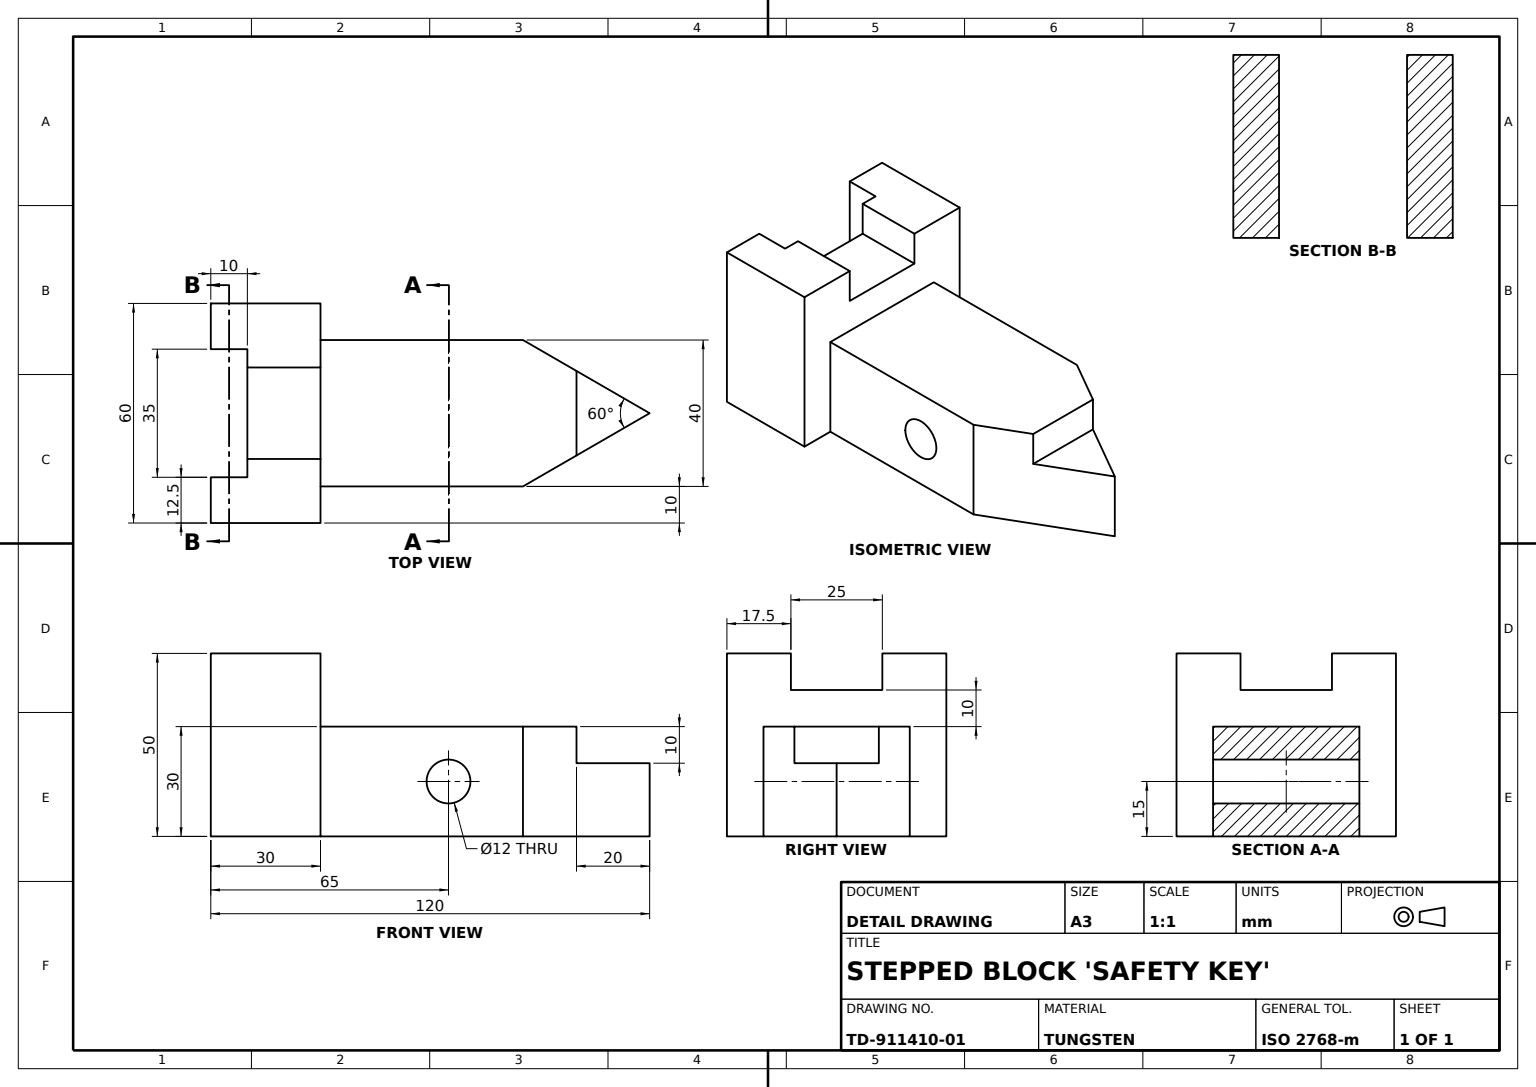
ISO-10303-21;
HEADER;
FILE_DESCRIPTION((''),'2;1');
FILE_NAME('','',(''),(''),'','','');
FILE_SCHEMA(('AUTOMOTIVE_DESIGN'));
ENDSEC;
DATA;
#1=APPLICATION_CONTEXT('');
#2=PRODUCT_CONTEXT('',#1,'mechanical');
#3=PRODUCT('','','',(#2));
#4=PRODUCT_DEFINITION_FORMATION('','',#3);
#5=PRODUCT_DEFINITION_CONTEXT('',#1,'design');
#6=PRODUCT_DEFINITION('','',#4,#5);
#7=PRODUCT_DEFINITION_SHAPE('','',#6);
#8=(LENGTH_UNIT()NAMED_UNIT(*)SI_UNIT(.MILLI.,.METRE.));
#9=(NAMED_UNIT(*)PLANE_ANGLE_UNIT()SI_UNIT($,.RADIAN.));
#10=(NAMED_UNIT(*)SI_UNIT($,.STERADIAN.)SOLID_ANGLE_UNIT());
#11=UNCERTAINTY_MEASURE_WITH_UNIT(LENGTH_MEASURE(0.005),#8,'distance_accuracy_value','');
#12=(GEOMETRIC_REPRESENTATION_CONTEXT(3)GLOBAL_UNCERTAINTY_ASSIGNED_CONTEXT((#11))GLOBAL_UNIT_ASSIGNED_CONTEXT((#8,#9,#10))REPRESENTATION_CONTEXT('',''));
#13=CARTESIAN_POINT('',(-5.,17.5,50.));
#14=VERTEX_POINT('',#13);
#15=CARTESIAN_POINT('',(-15.,17.5,50.));
#16=VERTEX_POINT('',#15);
#17=CARTESIAN_POINT('',(0.,17.5,50.));
#18=DIRECTION('',(-1.,0.,0.));
#19=VECTOR('',#18,1000.);
#20=LINE('',#17,#19);
#21=EDGE_CURVE('',#14,#16,#20,.T.);
#22=ORIENTED_EDGE('',*,*,#21,.F.);
#23=CARTESIAN_POINT('',(-5.,12.5,50.));
#24=VERTEX_POINT('',#23);
#25=CARTESIAN_POINT('',(-5.,0.,50.));
#26=DIRECTION('',(0.,1.,0.));
#27=VECTOR('',#26,1000.);
#28=LINE('',#25,#27);
#29=EDGE_CURVE('',#24,#14,#28,.T.);
#30=ORIENTED_EDGE('',*,*,#29,.F.);
#31=CARTESIAN_POINT('',(15.,12.5,50.));
#32=VERTEX_POINT('',#31);
#33=CARTESIAN_POINT('',(-30.,12.5,50.));
#34=DIRECTION('',(1.,0.,0.));
#35=VECTOR('',#34,1000.);
#36=LINE('',#33,#35);
#37=EDGE_CURVE('',#24,#32,#36,.T.);
#38=ORIENTED_EDGE('',*,*,#37,.T.);
#39=CARTESIAN_POINT('',(15.,30.,50.));
#40=VERTEX_POINT('',#39);
#41=CARTESIAN_POINT('',(15.,-30.,50.));
#42=LINE('',#41,#27);
#43=EDGE_CURVE('',#32,#40,#42,.T.);
#44=ORIENTED_EDGE('',*,*,#43,.T.);
#45=CARTESIAN_POINT('',(-15.,30.,50.));
#46=VERTEX_POINT('',#45);
#47=LINE('',#39,#19);
#48=EDGE_CURVE('',#40,#46,#47,.T.);
#49=ORIENTED_EDGE('',*,*,#48,.T.);
#50=DIRECTION('',(0.,-1.,0.));
#51=VECTOR('',#50,1000.);
#52=LINE('',#45,#51);
#53=EDGE_CURVE('',#46,#16,#52,.T.);
#54=ORIENTED_EDGE('',*,*,#53,.T.);
#55=EDGE_LOOP('',(#22,#30,#38,#44,#49,#54));
#56=FACE_BOUND('',#55,.T.);
#57=CARTESIAN_POINT('',(0.,0.,50.));
#58=DIRECTION('',(0.,0.,1.));
#59=AXIS2_PLACEMENT_3D('',#57,#58,#34);
#60=PLANE('',#59);
#61=ADVANCED_FACE('',(#56),#60,.T.);
#62=VERTEX_POINT('',#41);
#63=CARTESIAN_POINT('',(15.,-30.,0.));
#64=VERTEX_POINT('',#63);
#65=DIRECTION('',(0.,0.,-1.));
#66=VECTOR('',#65,1000.);
#67=LINE('',#41,#66);
#68=EDGE_CURVE('',#62,#64,#67,.T.);
#69=ORIENTED_EDGE('',*,*,#68,.F.);
#70=CARTESIAN_POINT('',(-15.,-30.,50.));
#71=VERTEX_POINT('',#70);
#72=LINE('',#70,#35);
#73=EDGE_CURVE('',#71,#62,#72,.T.);
#74=ORIENTED_EDGE('',*,*,#73,.F.);
#75=CARTESIAN_POINT('',(-15.,-30.,0.));
#76=VERTEX_POINT('',#75);
#77=LINE('',#70,#66);
#78=EDGE_CURVE('',#71,#76,#77,.T.);
#79=ORIENTED_EDGE('',*,*,#78,.T.);
#80=LINE('',#75,#35);
#81=EDGE_CURVE('',#76,#64,#80,.T.);
#82=ORIENTED_EDGE('',*,*,#81,.T.);
#83=EDGE_LOOP('',(#69,#74,#79,#82));
#84=FACE_BOUND('',#83,.T.);
#85=AXIS2_PLACEMENT_3D('',#70,#26,#58);
#86=PLANE('',#85);
#87=ADVANCED_FACE('',(#84),#86,.F.);
#88=CARTESIAN_POINT('',(-15.,-17.5,0.));
#89=VERTEX_POINT('',#88);
#90=CARTESIAN_POINT('',(-15.,30.,0.));
#91=LINE('',#90,#51);
#92=EDGE_CURVE('',#89,#76,#91,.T.);
#93=ORIENTED_EDGE('',*,*,#92,.T.);
#94=ORIENTED_EDGE('',*,*,#78,.F.);
#95=CARTESIAN_POINT('',(-15.,-17.5,50.));
#96=VERTEX_POINT('',#95);
#97=EDGE_CURVE('',#96,#71,#52,.T.);
#98=ORIENTED_EDGE('',*,*,#97,.F.);
#99=CARTESIAN_POINT('',(-15.,-17.5,62.));
#100=LINE('',#99,#66);
#101=EDGE_CURVE('',#96,#89,#100,.T.);
#102=ORIENTED_EDGE('',*,*,#101,.T.);
#103=EDGE_LOOP('',(#93,#94,#98,#102));
#104=FACE_BOUND('',#103,.T.);
#105=AXIS2_PLACEMENT_3D('',#45,#34,#65);
#106=PLANE('',#105);
#107=ADVANCED_FACE('',(#104),#106,.F.);
#108=CARTESIAN_POINT('',(44.,-20.,15.));
#109=VERTEX_POINT('',#108);
#110=CARTESIAN_POINT('',(50.,-20.,15.));
#111=AXIS2_PLACEMENT_3D('',#110,#26,#18);
#112=CIRCLE('',#111,6.);
#113=EDGE_CURVE('',#109,#109,#112,.T.);
#114=ORIENTED_EDGE('',*,*,#113,.F.);
#115=EDGE_LOOP('',(#114));
#116=FACE_BOUND('',#115,.T.);
#117=CARTESIAN_POINT('',(44.,20.,15.));
#118=VERTEX_POINT('',#117);
#119=CARTESIAN_POINT('',(50.,20.,15.));
#120=AXIS2_PLACEMENT_3D('',#119,#26,#18);
#121=CIRCLE('',#120,6.);
#122=EDGE_CURVE('',#118,#118,#121,.T.);
#123=ORIENTED_EDGE('',*,*,#122,.T.);
#124=EDGE_LOOP('',(#123));
#125=FACE_BOUND('',#124,.T.);
#126=CYLINDRICAL_SURFACE('',#111,6.);
#127=ADVANCED_FACE('',(#116,#125),#126,.F.);
#128=CARTESIAN_POINT('',(15.,20.,0.));
#129=VERTEX_POINT('',#128);
#130=CARTESIAN_POINT('',(70.358984,20.,0.));
#131=VERTEX_POINT('',#130);
#132=LINE('',#128,#35);
#133=EDGE_CURVE('',#129,#131,#132,.T.);
#134=ORIENTED_EDGE('',*,*,#133,.F.);
#135=CARTESIAN_POINT('',(15.,20.,30.));
#136=VERTEX_POINT('',#135);
#137=LINE('',#135,#66);
#138=EDGE_CURVE('',#136,#129,#137,.T.);
#139=ORIENTED_EDGE('',*,*,#138,.F.);
#140=CARTESIAN_POINT('',(70.358984,20.,30.));
#141=VERTEX_POINT('',#140);
#142=LINE('',#135,#35);
#143=EDGE_CURVE('',#136,#141,#142,.T.);
#144=ORIENTED_EDGE('',*,*,#143,.T.);
#145=CARTESIAN_POINT('',(70.358984,20.,62.));
#146=LINE('',#145,#66);
#147=EDGE_CURVE('',#141,#131,#146,.T.);
#148=ORIENTED_EDGE('',*,*,#147,.T.);
#149=EDGE_LOOP('',(#134,#139,#144,#148));
#150=FACE_BOUND('',#149,.T.);
#151=ORIENTED_EDGE('',*,*,#122,.F.);
#152=EDGE_LOOP('',(#151));
#153=FACE_BOUND('',#152,.T.);
#154=AXIS2_PLACEMENT_3D('',#135,#26,#18);
#155=PLANE('',#154);
#156=ADVANCED_FACE('',(#150,#153),#155,.T.);
#157=CARTESIAN_POINT('',(15.,30.,0.));
#158=VERTEX_POINT('',#157);
#159=LINE('',#39,#66);
#160=EDGE_CURVE('',#40,#158,#159,.T.);
#161=ORIENTED_EDGE('',*,*,#160,.T.);
#162=VERTEX_POINT('',#90);
#163=LINE('',#157,#19);
#164=EDGE_CURVE('',#158,#162,#163,.T.);
#165=ORIENTED_EDGE('',*,*,#164,.T.);
#166=LINE('',#45,#66);
#167=EDGE_CURVE('',#46,#162,#166,.T.);
#168=ORIENTED_EDGE('',*,*,#167,.F.);
#169=ORIENTED_EDGE('',*,*,#48,.F.);
#170=EDGE_LOOP('',(#161,#165,#168,#169));
#171=FACE_BOUND('',#170,.T.);
#172=AXIS2_PLACEMENT_3D('',#39,#50,#65);
#173=PLANE('',#172);
#174=ADVANCED_FACE('',(#171),#173,.F.);
#175=ORIENTED_EDGE('',*,*,#143,.F.);
#176=CARTESIAN_POINT('',(15.,-20.,30.));
#177=VERTEX_POINT('',#176);
#178=LINE('',#176,#27);
#179=EDGE_CURVE('',#177,#136,#178,.T.);
#180=ORIENTED_EDGE('',*,*,#179,.F.);
#181=CARTESIAN_POINT('',(70.358984,-20.,30.));
#182=VERTEX_POINT('',#181);
#183=CARTESIAN_POINT('',(105.,-20.,30.));
#184=LINE('',#183,#19);
#185=EDGE_CURVE('',#182,#177,#184,.T.);
#186=ORIENTED_EDGE('',*,*,#185,.F.);
#187=CARTESIAN_POINT('',(85.,-11.547005,30.));
#188=VERTEX_POINT('',#187);
#189=CARTESIAN_POINT('',(26.25,-45.466334,30.));
#190=DIRECTION('',(-0.866025404,-0.5,0.));
#191=VECTOR('',#190,1000.);
#192=LINE('',#189,#191);
#193=EDGE_CURVE('',#188,#182,#192,.T.);
#194=ORIENTED_EDGE('',*,*,#193,.F.);
#195=CARTESIAN_POINT('',(85.,11.547005,30.));
#196=VERTEX_POINT('',#195);
#197=CARTESIAN_POINT('',(85.,0.,30.));
#198=LINE('',#197,#51);
#199=EDGE_CURVE('',#196,#188,#198,.T.);
#200=ORIENTED_EDGE('',*,*,#199,.F.);
#201=CARTESIAN_POINT('',(26.25,45.466334,30.));
#202=DIRECTION('',(-0.866025404,0.5,0.));
#203=VECTOR('',#202,1000.);
#204=LINE('',#201,#203);
#205=EDGE_CURVE('',#196,#141,#204,.T.);
#206=ORIENTED_EDGE('',*,*,#205,.T.);
#207=EDGE_LOOP('',(#175,#180,#186,#194,#200,#206));
#208=FACE_BOUND('',#207,.T.);
#209=CARTESIAN_POINT('',(0.,0.,30.));
#210=AXIS2_PLACEMENT_3D('',#209,#65,#18);
#211=PLANE('',#210);
#212=ADVANCED_FACE('',(#208),#211,.F.);
#213=CARTESIAN_POINT('',(70.358984,-20.,0.));
#214=VERTEX_POINT('',#213);
#215=CARTESIAN_POINT('',(70.358984,-20.,62.));
#216=LINE('',#215,#66);
#217=EDGE_CURVE('',#182,#214,#216,.T.);
#218=ORIENTED_EDGE('',*,*,#217,.F.);
#219=ORIENTED_EDGE('',*,*,#185,.T.);
#220=CARTESIAN_POINT('',(15.,-20.,0.));
#221=VERTEX_POINT('',#220);
#222=LINE('',#176,#66);
#223=EDGE_CURVE('',#177,#221,#222,.T.);
#224=ORIENTED_EDGE('',*,*,#223,.T.);
#225=CARTESIAN_POINT('',(105.,-20.,0.));
#226=LINE('',#225,#19);
#227=EDGE_CURVE('',#214,#221,#226,.T.);
#228=ORIENTED_EDGE('',*,*,#227,.F.);
#229=EDGE_LOOP('',(#218,#219,#224,#228));
#230=FACE_BOUND('',#229,.T.);
#231=ORIENTED_EDGE('',*,*,#113,.T.);
#232=EDGE_LOOP('',(#231));
#233=FACE_BOUND('',#232,.T.);
#234=AXIS2_PLACEMENT_3D('',#183,#50,#34);
#235=PLANE('',#234);
#236=ADVANCED_FACE('',(#230,#233),#235,.T.);
#237=CARTESIAN_POINT('',(85.,-11.547005,20.));
#238=VERTEX_POINT('',#237);
#239=CARTESIAN_POINT('',(85.,-11.547005,62.));
#240=VECTOR('',#58,1000.);
#241=LINE('',#239,#240);
#242=EDGE_CURVE('',#238,#188,#241,.T.);
#243=ORIENTED_EDGE('',*,*,#242,.F.);
#244=CARTESIAN_POINT('',(85.,11.547005,20.));
#245=VERTEX_POINT('',#244);
#246=CARTESIAN_POINT('',(85.,15.,20.));
#247=LINE('',#246,#51);
#248=EDGE_CURVE('',#238,#245,#247,.F.);
#249=ORIENTED_EDGE('',*,*,#248,.T.);
#250=CARTESIAN_POINT('',(85.,11.547005,62.));
#251=LINE('',#250,#240);
#252=EDGE_CURVE('',#245,#196,#251,.T.);
#253=ORIENTED_EDGE('',*,*,#252,.T.);
#254=ORIENTED_EDGE('',*,*,#199,.T.);
#255=EDGE_LOOP('',(#243,#249,#253,#254));
#256=FACE_BOUND('',#255,.T.);
#257=CARTESIAN_POINT('',(85.,15.,44.));
#258=AXIS2_PLACEMENT_3D('',#257,#34,#65);
#259=PLANE('',#258);
#260=ADVANCED_FACE('',(#256),#259,.T.);
#261=ORIENTED_EDGE('',*,*,#101,.F.);
#262=CARTESIAN_POINT('',(-5.,-17.5,50.));
#263=VERTEX_POINT('',#262);
#264=CARTESIAN_POINT('',(0.,-17.5,50.));
#265=LINE('',#264,#35);
#266=EDGE_CURVE('',#96,#263,#265,.T.);
#267=ORIENTED_EDGE('',*,*,#266,.T.);
#268=CARTESIAN_POINT('',(-5.,-17.5,0.));
#269=VERTEX_POINT('',#268);
#270=CARTESIAN_POINT('',(-5.,-17.5,62.));
#271=LINE('',#270,#66);
#272=EDGE_CURVE('',#269,#263,#271,.F.);
#273=ORIENTED_EDGE('',*,*,#272,.F.);
#274=CARTESIAN_POINT('',(0.,-17.5,0.));
#275=LINE('',#274,#19);
#276=EDGE_CURVE('',#269,#89,#275,.T.);
#277=ORIENTED_EDGE('',*,*,#276,.T.);
#278=EDGE_LOOP('',(#261,#267,#273,#277));
#279=FACE_BOUND('',#278,.T.);
#280=AXIS2_PLACEMENT_3D('',#270,#50,#65);
#281=PLANE('',#280);
#282=ADVANCED_FACE('',(#279),#281,.F.);
#283=CARTESIAN_POINT('',(-15.,17.5,0.));
#284=VERTEX_POINT('',#283);
#285=CARTESIAN_POINT('',(-5.,17.5,0.));
#286=VERTEX_POINT('',#285);
#287=CARTESIAN_POINT('',(0.,17.5,0.));
#288=LINE('',#287,#35);
#289=EDGE_CURVE('',#284,#286,#288,.T.);
#290=ORIENTED_EDGE('',*,*,#289,.T.);
#291=CARTESIAN_POINT('',(-5.,17.5,62.));
#292=LINE('',#291,#66);
#293=EDGE_CURVE('',#286,#14,#292,.F.);
#294=ORIENTED_EDGE('',*,*,#293,.T.);
#295=ORIENTED_EDGE('',*,*,#21,.T.);
#296=CARTESIAN_POINT('',(-15.,17.5,62.));
#297=LINE('',#296,#66);
#298=EDGE_CURVE('',#16,#284,#297,.T.);
#299=ORIENTED_EDGE('',*,*,#298,.T.);
#300=EDGE_LOOP('',(#290,#294,#295,#299));
#301=FACE_BOUND('',#300,.T.);
#302=AXIS2_PLACEMENT_3D('',#296,#26,#58);
#303=PLANE('',#302);
#304=ADVANCED_FACE('',(#301),#303,.F.);
#305=CARTESIAN_POINT('',(15.,12.5,40.));
#306=VERTEX_POINT('',#305);
#307=LINE('',#31,#240);
#308=EDGE_CURVE('',#306,#32,#307,.T.);
#309=ORIENTED_EDGE('',*,*,#308,.T.);
#310=ORIENTED_EDGE('',*,*,#37,.F.);
#311=CARTESIAN_POINT('',(-5.,12.5,40.));
#312=VERTEX_POINT('',#311);
#313=LINE('',#23,#240);
#314=EDGE_CURVE('',#312,#24,#313,.T.);
#315=ORIENTED_EDGE('',*,*,#314,.F.);
#316=CARTESIAN_POINT('',(-30.,12.5,40.));
#317=LINE('',#316,#35);
#318=EDGE_CURVE('',#306,#312,#317,.F.);
#319=ORIENTED_EDGE('',*,*,#318,.F.);
#320=EDGE_LOOP('',(#309,#310,#315,#319));
#321=FACE_BOUND('',#320,.T.);
#322=AXIS2_PLACEMENT_3D('',#33,#50,#65);
#323=PLANE('',#322);
#324=ADVANCED_FACE('',(#321),#323,.T.);
#325=ORIENTED_EDGE('',*,*,#308,.F.);
#326=CARTESIAN_POINT('',(15.,-12.5,40.));
#327=VERTEX_POINT('',#326);
#328=CARTESIAN_POINT('',(15.,-30.,40.));
#329=LINE('',#328,#27);
#330=EDGE_CURVE('',#327,#306,#329,.T.);
#331=ORIENTED_EDGE('',*,*,#330,.F.);
#332=CARTESIAN_POINT('',(15.,-12.5,50.));
#333=VERTEX_POINT('',#332);
#334=LINE('',#332,#66);
#335=EDGE_CURVE('',#333,#327,#334,.T.);
#336=ORIENTED_EDGE('',*,*,#335,.F.);
#337=EDGE_CURVE('',#62,#333,#42,.T.);
#338=ORIENTED_EDGE('',*,*,#337,.F.);
#339=ORIENTED_EDGE('',*,*,#68,.T.);
#340=LINE('',#63,#27);
#341=EDGE_CURVE('',#64,#221,#340,.T.);
#342=ORIENTED_EDGE('',*,*,#341,.T.);
#343=ORIENTED_EDGE('',*,*,#223,.F.);
#344=ORIENTED_EDGE('',*,*,#179,.T.);
#345=ORIENTED_EDGE('',*,*,#138,.T.);
#346=EDGE_CURVE('',#129,#158,#340,.T.);
#347=ORIENTED_EDGE('',*,*,#346,.T.);
#348=ORIENTED_EDGE('',*,*,#160,.F.);
#349=ORIENTED_EDGE('',*,*,#43,.F.);
#350=EDGE_LOOP('',(#325,#331,#336,#338,#339,#342,#343,#344,#345,#347,#348,#349));
#351=FACE_BOUND('',#350,.T.);
#352=AXIS2_PLACEMENT_3D('',#41,#18,#58);
#353=PLANE('',#352);
#354=ADVANCED_FACE('',(#351),#353,.F.);
#355=CARTESIAN_POINT('',(-5.,-12.5,50.));
#356=VERTEX_POINT('',#355);
#357=CARTESIAN_POINT('',(-30.,-12.5,50.));
#358=LINE('',#357,#35);
#359=EDGE_CURVE('',#356,#333,#358,.T.);
#360=ORIENTED_EDGE('',*,*,#359,.F.);
#361=EDGE_CURVE('',#263,#356,#28,.T.);
#362=ORIENTED_EDGE('',*,*,#361,.F.);
#363=ORIENTED_EDGE('',*,*,#266,.F.);
#364=ORIENTED_EDGE('',*,*,#97,.T.);
#365=ORIENTED_EDGE('',*,*,#73,.T.);
#366=ORIENTED_EDGE('',*,*,#337,.T.);
#367=EDGE_LOOP('',(#360,#362,#363,#364,#365,#366));
#368=FACE_BOUND('',#367,.T.);
#369=ADVANCED_FACE('',(#368),#60,.T.);
#370=EDGE_CURVE('',#162,#284,#91,.T.);
#371=ORIENTED_EDGE('',*,*,#370,.F.);
#372=ORIENTED_EDGE('',*,*,#164,.F.);
#373=ORIENTED_EDGE('',*,*,#346,.F.);
#374=ORIENTED_EDGE('',*,*,#133,.T.);
#375=CARTESIAN_POINT('',(105.,0.,0.));
#376=VERTEX_POINT('',#375);
#377=CARTESIAN_POINT('',(26.25,45.466334,0.));
#378=LINE('',#377,#203);
#379=EDGE_CURVE('',#376,#131,#378,.T.);
#380=ORIENTED_EDGE('',*,*,#379,.F.);
#381=CARTESIAN_POINT('',(26.25,-45.466334,0.));
#382=LINE('',#381,#191);
#383=EDGE_CURVE('',#376,#214,#382,.T.);
#384=ORIENTED_EDGE('',*,*,#383,.T.);
#385=ORIENTED_EDGE('',*,*,#227,.T.);
#386=ORIENTED_EDGE('',*,*,#341,.F.);
#387=ORIENTED_EDGE('',*,*,#81,.F.);
#388=ORIENTED_EDGE('',*,*,#92,.F.);
#389=ORIENTED_EDGE('',*,*,#276,.F.);
#390=CARTESIAN_POINT('',(-5.,0.,0.));
#391=LINE('',#390,#51);
#392=EDGE_CURVE('',#286,#269,#391,.T.);
#393=ORIENTED_EDGE('',*,*,#392,.F.);
#394=ORIENTED_EDGE('',*,*,#289,.F.);
#395=EDGE_LOOP('',(#371,#372,#373,#374,#380,#384,#385,#386,#387,#388,#389,#393,#394));
#396=FACE_BOUND('',#395,.T.);
#397=CARTESIAN_POINT('',(0.,0.,0.));
#398=AXIS2_PLACEMENT_3D('',#397,#65,#18);
#399=PLANE('',#398);
#400=ADVANCED_FACE('',(#396),#399,.T.);
#401=ORIENTED_EDGE('',*,*,#217,.T.);
#402=ORIENTED_EDGE('',*,*,#383,.F.);
#403=CARTESIAN_POINT('',(105.,0.,20.));
#404=VERTEX_POINT('',#403);
#405=CARTESIAN_POINT('',(105.,0.,62.));
#406=LINE('',#405,#66);
#407=EDGE_CURVE('',#404,#376,#406,.T.);
#408=ORIENTED_EDGE('',*,*,#407,.F.);
#409=LINE('',#403,#191);
#410=EDGE_CURVE('',#404,#238,#409,.T.);
#411=ORIENTED_EDGE('',*,*,#410,.T.);
#412=ORIENTED_EDGE('',*,*,#242,.T.);
#413=ORIENTED_EDGE('',*,*,#193,.T.);
#414=EDGE_LOOP('',(#401,#402,#408,#411,#412,#413));
#415=FACE_BOUND('',#414,.T.);
#416=DIRECTION('',(0.5,-0.866025404,0.));
#417=DIRECTION('',(0.866025404,0.5,0.));
#418=AXIS2_PLACEMENT_3D('',#405,#416,#417);
#419=PLANE('',#418);
#420=ADVANCED_FACE('',(#415),#419,.T.);
#421=ORIENTED_EDGE('',*,*,#330,.T.);
#422=ORIENTED_EDGE('',*,*,#318,.T.);
#423=CARTESIAN_POINT('',(-5.,-12.5,40.));
#424=VERTEX_POINT('',#423);
#425=LINE('',#311,#27);
#426=EDGE_CURVE('',#424,#312,#425,.T.);
#427=ORIENTED_EDGE('',*,*,#426,.F.);
#428=CARTESIAN_POINT('',(-30.,-12.5,40.));
#429=LINE('',#428,#35);
#430=EDGE_CURVE('',#327,#424,#429,.F.);
#431=ORIENTED_EDGE('',*,*,#430,.F.);
#432=EDGE_LOOP('',(#421,#422,#427,#431));
#433=FACE_BOUND('',#432,.T.);
#434=AXIS2_PLACEMENT_3D('',#316,#58,#34);
#435=PLANE('',#434);
#436=ADVANCED_FACE('',(#433),#435,.T.);
#437=ORIENTED_EDGE('',*,*,#252,.F.);
#438=LINE('',#403,#203);
#439=EDGE_CURVE('',#404,#245,#438,.T.);
#440=ORIENTED_EDGE('',*,*,#439,.F.);
#441=ORIENTED_EDGE('',*,*,#407,.T.);
#442=ORIENTED_EDGE('',*,*,#379,.T.);
#443=ORIENTED_EDGE('',*,*,#147,.F.);
#444=ORIENTED_EDGE('',*,*,#205,.F.);
#445=EDGE_LOOP('',(#437,#440,#441,#442,#443,#444));
#446=FACE_BOUND('',#445,.T.);
#447=DIRECTION('',(-0.5,-0.866025404,0.));
#448=DIRECTION('',(0.866025404,-0.5,0.));
#449=AXIS2_PLACEMENT_3D('',#405,#447,#448);
#450=PLANE('',#449);
#451=ADVANCED_FACE('',(#446),#450,.F.);
#452=ORIENTED_EDGE('',*,*,#370,.T.);
#453=ORIENTED_EDGE('',*,*,#298,.F.);
#454=ORIENTED_EDGE('',*,*,#53,.F.);
#455=ORIENTED_EDGE('',*,*,#167,.T.);
#456=EDGE_LOOP('',(#452,#453,#454,#455));
#457=FACE_BOUND('',#456,.T.);
#458=ADVANCED_FACE('',(#457),#106,.F.);
#459=ORIENTED_EDGE('',*,*,#430,.T.);
#460=LINE('',#423,#66);
#461=EDGE_CURVE('',#356,#424,#460,.T.);
#462=ORIENTED_EDGE('',*,*,#461,.F.);
#463=ORIENTED_EDGE('',*,*,#359,.T.);
#464=ORIENTED_EDGE('',*,*,#335,.T.);
#465=EDGE_LOOP('',(#459,#462,#463,#464));
#466=FACE_BOUND('',#465,.T.);
#467=AXIS2_PLACEMENT_3D('',#428,#26,#58);
#468=PLANE('',#467);
#469=ADVANCED_FACE('',(#466),#468,.T.);
#470=ORIENTED_EDGE('',*,*,#248,.F.);
#471=ORIENTED_EDGE('',*,*,#410,.F.);
#472=ORIENTED_EDGE('',*,*,#439,.T.);
#473=EDGE_LOOP('',(#470,#471,#472));
#474=FACE_BOUND('',#473,.T.);
#475=CARTESIAN_POINT('',(0.,0.,20.));
#476=AXIS2_PLACEMENT_3D('',#475,#58,#34);
#477=PLANE('',#476);
#478=ADVANCED_FACE('',(#474),#477,.T.);
#479=ORIENTED_EDGE('',*,*,#29,.T.);
#480=ORIENTED_EDGE('',*,*,#293,.F.);
#481=ORIENTED_EDGE('',*,*,#392,.T.);
#482=ORIENTED_EDGE('',*,*,#272,.T.);
#483=ORIENTED_EDGE('',*,*,#361,.T.);
#484=ORIENTED_EDGE('',*,*,#461,.T.);
#485=ORIENTED_EDGE('',*,*,#426,.T.);
#486=ORIENTED_EDGE('',*,*,#314,.T.);
#487=EDGE_LOOP('',(#479,#480,#481,#482,#483,#484,#485,#486));
#488=FACE_BOUND('',#487,.T.);
#489=AXIS2_PLACEMENT_3D('',#291,#34,#65);
#490=PLANE('',#489);
#491=ADVANCED_FACE('',(#488),#490,.F.);
#492=CLOSED_SHELL('',(#61,#87,#107,#127,#156,#174,#212,#236,#260,#282,#304,#324,#354,#369,#400,#420,#436,#451,#458,#469,#478,#491));
#493=MANIFOLD_SOLID_BREP('',#492);
#494=ADVANCED_BREP_SHAPE_REPRESENTATION('',(#493),#12);
#495=SHAPE_DEFINITION_REPRESENTATION(#7,#494);
ENDSEC;
END-ISO-10303-21;
